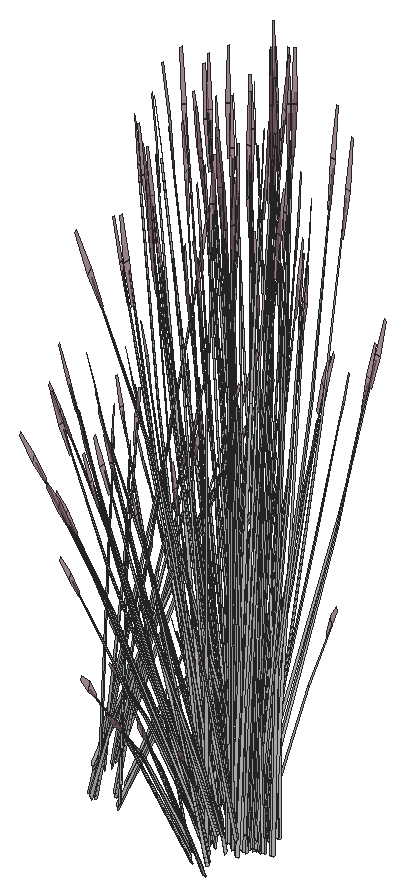
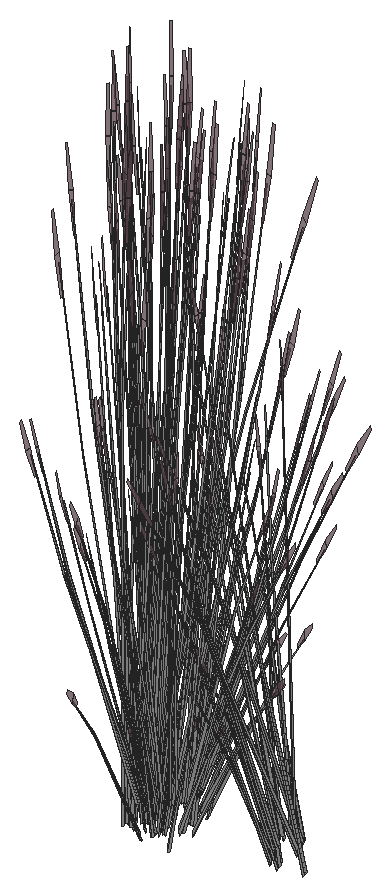
# SketchUp Ruby script. Lengths in inches.
U = 1.inch
M = Sketchup.active_model
def pt(a) = Geom::Point3d.new(a.map { |v| v * U })
def face(e, loops, mat)
  f = e.add_face(loops[0].map { |a| pt(a) })
  loops[1..].each { |l| e.add_face(l.map { |a| pt(a) }).erase! }
  f.material = f.back_material = mat if mat
  f
end
# faces: each face lists its corners as indices into pts; further lists are holes
def faces(e, pts, list, mat = nil) = list.each { |f| face(e, (f[0].is_a?(Array) ? f : [f]).map { |l| l.map { |i| pts[i] } }, mat) }
# xy, xz, yz: faces in a plane at the given z, y or x. An outline is a flat list of corners, or four numbers for a rectangle; further outlines are holes
def ring(l) = l.size == 4 ? [[l[0], l[1]], [l[2], l[1]], [l[2], l[3]], [l[0], l[3]]] : l.each_slice(2).to_a
def flat(e, list, mat, &to3) = list.each { |f| face(e, (f[0].is_a?(Array) ? f : [f]).map { |l| ring(l).map { |u, v| to3.(u, v) } }, mat) }
def xy(e, z, list, mat = nil) = flat(e, list, mat) { |x, y| [x, y, z] }
def xz(e, y, list, mat = nil) = flat(e, list, mat) { |x, z| [x, y, z] }
def yz(e, x, list, mat = nil) = flat(e, list, mat) { |y, z| [x, y, z] }
def lines(e, pts, list) = list.each { |a, b| e.add_line(pt(pts[a]), pt(pts[b])) }
# prism: a flat outline (further loops are holes) pulled along v
def prism(e, loops, v, mat = nil)
  f = face(e, loops, mat); d = Geom::Vector3d.new(v.map { |x| x * U })
  f.pushpull(f.normal.samedirection?(d) ? d.length : -d.length)
end
def box(e, o, s, mat = nil) = prism(e, [[o, [o[0] + s[0], o[1], o[2]], [o[0] + s[0], o[1] + s[1], o[2]], [o[0], o[1] + s[1], o[2]]]], [0, 0, s[2]], mat)
def at(x, y, z, deg = 0) = Geom::Transformation.translation(pt([x, y, z])) * Geom::Transformation.rotation(ORIGIN, Z_AXIS, deg.degrees)
def axes(o, x, y, z) = Geom::Transformation.new([*x, 0, *y, 0, *z, 0, *pt(o).to_a, 1])
def part(name) = M.definitions.add(name)
# library, detail: a bought-in or finely detailed component or shape, given as its bounding box
def library(name, o, s) = part(name).tap { |d| box(d.entities, o, s) }
def detail(e, o, s) = box(e.add_group.entities, o, s)
def put(e, d, t, mat = nil) = e.add_instance(d, t).tap { |i| i.material = mat if mat }
def group(e, t, mat = nil) = e.add_group.tap { |g| g.transformation = t; g.material = mat if mat }.entities
root = M.entities
M.materials.add("LightPink_Translucent").color = [144, 107, 117]
M.materials["LightPink_Translucent"].alpha = 0.75
M.materials.add("[_0053_Ivory_]").color = [200, 200, 200]
c1 = part("blade")
p = [[2.15,0.21,22],[0,0.17,0],[0.09,0.45,0],[2.18,0.31,22],[2.29,0.31,22],[0.38,0.45,0],
  [2.48,0.24,33],[2.49,0.24,33],[2.48,0.22,33]]
faces(c1.entities,p,[[0,1,2,3],[4,5,2,3],[6,3,4,7],[8,0,3,6]])
c2 = part("seeds")
p = [[0.3,-0.1,1.38],[-0.01,-0.03,1.59],[-0.01,-0.03,0.03],[0.14,-0.07,-0.07],[0.29,-0.03,3],[0.15,0.01,3.11]]
faces(c2.entities,p,[[0,1,2,3],[1,0,4,5]],"LightPink_Translucent")
c3 = part("blade with seeds")
put(c3.entities,c1,at(0,0,0))
put(c3.entities,c2,axes([2.4,0.25,30.99],[1.5799,-0.05474,1.17369],[-0.12525,1.92788,0.29478],[-0.07173,-0.02425,1.56792]))
put(root,c3,axes([471.34,101.96,128.71],[0.63179,0.1031,-0.62353],[-0.13332,0.63596,-0.16365],[0.18854,0.07706,1.37633]),"[_0053_Ivory_]")
put(root,c3,axes([481.84,101.41,130.53],[0.25192,-0.01424,1.71376],[-0.16712,0.61729,0.13857],[-0.35901,-0.03818,0.73262]),"[_0053_Ivory_]")
put(root,c3,axes([474.03,102.33,128.91],[-0.37654,-0.40212,-0.06488],[0.4124,-0.36845,-0.29416],[0.11685,-0.02594,0.97024]),"[_0053_Ivory_]")
put(root,c3,axes([473.17,100.29,129.42],[-0.2023,0.32011,1.1486],[-0.17388,-0.43009,0.84392],[0.16708,-0.10777,0.25299]),"[_0053_Ivory_]")
put(root,c3,axes([471.21,103.32,130.53],[-0.2256,-0.10835,1.71376],[0.46687,-0.45453,0.13857],[0.29098,0.20505,0.73262]),"[_0053_Ivory_]")
put(root,c3,axes([481.95,102.5,130.53],[0.21074,-0.13302,1.71376],[0.17741,0.61464,0.13857],[-0.33083,0.13891,0.73262]),"[_0053_Ivory_]")
put(root,c3,axes([472.88,101.49,131.18],[0.52868,-0.08987,-0.35414],[0.1396,0.51376,0.4572],[0.1515,-0.13799,0.87481]),"[_0053_Ivory_]")
put(root,c3,axes([481.29,103.54,129.24],[0.21107,0.05162,1.43002],[0.13604,0.52729,-0.30754],[-0.28671,0.0987,0.61141]),"[_0053_Ivory_]")
put(root,c3,axes([472.46,101.66,131.63],[0.31725,-0.49618,-0.71045],[0.55593,0.35263,0.08574],[0.18942,-0.17977,1.00501]),"[_0053_Ivory_]")
put(root,c3,axes([472.45,104.33,131.18],[0.34557,0.39372,-0.35414],[-0.39459,0.37271,0.4572],[0.20048,0.05671,0.87481]),"[_0053_Ivory_]")
put(root,c3,axes([483.16,101.86,130],[0.17264,-0.09097,1.77064],[0.05953,0.63516,0.13857],[-0.37394,0.08428,0.63284]),"[_0053_Ivory_]")
put(root,c3,axes([482.6,100.84,131.63],[-0.60713,-0.01514,-0.71045],[0.04078,-0.63759,0.08574],[-0.25721,-0.06729,1.00501]),"[_0053_Ivory_]")
put(root,c3,axes([482.11,100.99,129.24],[0.11858,0.17508,1.43002],[-0.27325,0.4759,-0.30754],[-0.28057,-0.11375,0.61141]),"[_0053_Ivory_]")
put(root,c3,axes([472.72,102.71,131.33],[0.16454,-0.57202,-0.51099],[0.56413,0.19607,-0.3958],[0.22713,-0.05245,0.97773]),"[_0053_Ivory_]")
put(root,c3,axes([474.14,103.07,129.42],[-0.37526,0.10382,1.1486],[0.17664,-0.42906,0.84392],[0.19907,0.02936,0.25299]),"[_0053_Ivory_]")
put(root,c3,axes([481.625,101.94,131.18],[-0.50475,-0.17543,-0.35414],[0.14722,-0.5118,0.4572],[-0.20322,0.04693,0.87481]),"[_0053_Ivory_]")
put(root,c3,axes([482.32,100.42,130.53],[0.2256,0.10835,1.71376],[-0.46687,0.45453,0.13857],[-0.29098,-0.20505,0.73262]),"[_0053_Ivory_]")
put(root,c3,axes([472.92,101.21,129.24],[-0.21697,-0.01863,1.43002],[-0.22228,-0.49966,-0.30754],[0.26655,-0.14135,0.61141]),"[_0053_Ivory_]")
put(root,c3,axes([473.06,102.97,131.18],[0.50475,0.17543,-0.35414],[-0.14722,0.5118,0.4572],[0.20322,-0.04693,0.87481]),"[_0053_Ivory_]")
put(root,c3,axes([481.97,102.2,131.33],[-0.16454,0.57202,-0.51099],[-0.56413,-0.19607,-0.3958],[-0.22713,0.05245,0.97773]),"[_0053_Ivory_]")
put(root,c3,axes([472.09,104.07,131.63],[0.60713,0.01514,-0.71045],[-0.04078,0.63759,0.08574],[0.25721,0.06729,1.00501]),"[_0053_Ivory_]")
put(root,c3,axes([482.4,100.97,131.33],[-0.44101,0.41656,-0.51099],[-0.38623,-0.44004,-0.3958],[-0.22407,-0.06338,0.97773]),"[_0053_Ivory_]")
put(root,c3,axes([481.6875,102.17,128.15],[0.0154,0.09911,1.76342],[-0.31051,0.51756,-0.26939],[-0.22056,-0.02609,0.30037]),"[_0053_Ivory_]")
put(root,c3,axes([473.32,102.87,128.64],[-0.39118,0.07547,1.41583],[-0.06226,-0.6007,0.08104],[0.27398,-0.09092,0.80566]),"[_0053_Ivory_]")
put(root,c3,axes([473.75,102.47,128.15],[-0.03174,-0.09547,1.76342],[0.22015,-0.55846,-0.26939],[0.22208,-0.00803,0.30037]),"[_0053_Ivory_]")
put(root,c3,axes([471.6875,102.33,130.53],[-0.25192,0.01424,1.71376],[0.16712,-0.61729,0.13857],[0.35901,0.03818,0.73262]),"[_0053_Ivory_]")
put(root,c3,axes([480.85,104.65,129.42],[0.25312,-0.28501,1.1486],[0.09988,0.45119,0.84392],[-0.18292,0.08079,0.25299]),"[_0053_Ivory_]")
put(root,c3,axes([472.61,102.91,131.63],[0.53369,-0.27773,-0.71045],[0.29743,0.5717,0.08574],[0.25786,-0.06494,1.00501]),"[_0053_Ivory_]")
put(root,c3,axes([482.23,100.57,131.18],[-0.34557,-0.39372,-0.35414],[0.39459,-0.37271,0.4572],[-0.20048,-0.05671,0.87481]),"[_0053_Ivory_]")
put(root,c3,axes([482.72,102.91,130.53],[0.1517,-0.19322,1.71376],[0.38303,0.52154,0.13857],[-0.26271,0.23751,0.73262]),"[_0053_Ivory_]")
put(root,c3,axes([481.81,103.42,131.18],[-0.52868,0.08987,-0.35414],[-0.1396,-0.51376,0.4572],[-0.1515,0.13799,0.87481]),"[_0053_Ivory_]")
put(root,c3,axes([481.52,104.94,128.15],[0.08147,0.06283,1.76342],[0.13814,0.58211,-0.26939],[-0.18056,0.12413,0.30037]),"[_0053_Ivory_]")
put(root,c3,axes([481.4,101.52,129.42],[0.38775,-0.045,1.1486],[-0.24596,0.39648,0.84392],[-0.19161,-0.05948,0.25299]),"[_0053_Ivory_]")
put(root,c3,axes([473.43,103.76,129.24],[-0.14627,-0.15466,1.43002],[0.19032,-0.51164,-0.30754],[0.29594,0.06931,0.61141]),"[_0053_Ivory_]")
put(root,c3,axes([482.61,103.39,130.53],[0.11309,-0.21615,1.71376],[0.47441,0.44731,0.13857],[-0.21402,0.27879,0.73262]),"[_0053_Ivory_]")
put(root,c3,axes([482.24,103.48,131.33],[0.15602,0.5742,-0.51099],[-0.59087,0.10045,-0.3958],[-0.16933,0.15423,0.97773]),"[_0053_Ivory_]")
put(root,c3,axes([483.72,103.06,128.71],[-0.63179,-0.1031,-0.62353],[0.13332,-0.63596,-0.16365],[-0.18854,-0.07706,1.37633]),"[_0053_Ivory_]")
put(root,c3,axes([483.65,100.09,131.63],[-0.51789,-0.30395,-0.71045],[0.36805,-0.53263,0.08574],[-0.18764,-0.18149,1.00501]),"[_0053_Ivory_]")
put(root,c3,axes([483.41,100.1,131.33],[-0.59932,0.14948,-0.51099],[-0.10484,-0.56611,-0.3958],[-0.16097,-0.16223,0.97773]),"[_0053_Ivory_]")
put(root,c3,axes([482.89,104.27,128.67],[-0.56842,-0.31443,-0.49651],[0.33976,-0.56381,0],[-0.12946,-0.07161,1.57504]),"[_0053_Ivory_]")
put(root,c3,axes([482.64,99.59,128.15],[-0.05883,0.08284,1.76342],[-0.59454,0.17861,-0.26939],[-0.14363,-0.16248,0.30037]),"[_0053_Ivory_]")
put(root,c3,axes([483.23,104.65,129.03],[-0.37973,0.63014,0],[-0.6353,-0.35142,-0.51607],[-0.14469,-0.08004,1.63711]),"[_0053_Ivory_]")
put(root,c3,axes([482.54,105.5625,129.24],[0.19166,-0.0992,1.43002],[0.4732,0.29912,-0.30754],[-0.14084,0.25882,0.61141]),"[_0053_Ivory_]")
put(root,c3,axes([482.27,99.9,128.78],[-0.1752,0.51349,-0.03893],[-0.53924,-0.15795,-0.17649],[-0.08187,-0.08399,0.58215]),"[_0053_Ivory_]")
put(root,c3,axes([483.07,99.26,129.24],[-0.03678,0.20572,1.43002],[-0.53767,0.17221,-0.30754],[-0.12568,-0.26589,0.61141]),"[_0053_Ivory_]")
put(root,c3,axes([483.25,99.79,130.53],[0.13883,0.2019,1.71376],[-0.64153,0.16998,0.13857],[-0.14499,-0.31697,0.73262]),"[_0053_Ivory_]")
put(root,c3,axes([484.43,103.16,129.32],[-0.61322,0.4175,-0.29095],[-0.40778,-0.58992,-0.50002],[-0.1513,-0.05991,1.59708]),"[_0053_Ivory_]")
put(root,c3,axes([483.47,99.68,131.18],[-0.0938,-0.50652,-0.35414],[0.53623,-0.13375,0.4572],[-0.14403,-0.14515,0.87481]),"[_0053_Ivory_]")
put(root,c3,axes([481.98,102.25,129.03],[-0.75945,0,0],[0,-0.70283,-0.51607],[0,-0.16007,1.63711]),"[_0053_Ivory_]")
put(root,c3,axes([483.05,104.03,128.68],[-0.14267,-0.54795,-0.30978],[0.56663,-0.1556,0.30978],[-0.11423,-0.06319,1.38974]),"[_0053_Ivory_]")
put(root,c3,axes([482.74,104.61,131.18],[-0.41095,0.33109,-0.35414],[-0.38901,-0.37805,0.4572],[-0.05919,0.19208,0.87481]),"[_0053_Ivory_]")
put(root,c3,axes([484.84,103.61,128.71],[-0.40909,0.47266,-0.62353],[-0.50819,-0.4286,-0.16365],[-0.16393,0.11791,1.37633]),"[_0053_Ivory_]")
put(root,c3,axes([482.57,102.0625,128.98],[-0.56493,0.5287,0.30756],[-0.56528,-0.52313,-0.36492],[-0.01973,-0.15014,1.64885]),"[_0053_Ivory_]")
put(root,c3,axes([484.89,103.52,129.98],[0.52485,0.25358,1.51261],[-0.51417,0.54629,0.59816],[-0.23031,-0.32378,1.26806]),"[_0053_Ivory_]")
put(root,c3,axes([482.89,98.93,129.42],[0.31682,0.21887,1.1486],[-0.4614,0.13157,0.84392],[-0.09872,-0.16821,0.25299]),"[_0053_Ivory_]")
put(root,c3,axes([485.12,103.35,129.12],[-0.59306,-0.50614,-0.25192],[0.49904,-0.56836,0.5513],[-0.1597,0.05921,1.68216]),"[_0053_Ivory_]")
put(root,c3,axes([484.04,102.86,128.86],[-0.36485,-0.52782,-0.44739],[0.55265,-0.37168,0.21531],[-0.11807,-0.06531,1.43643]),"[_0053_Ivory_]")
put(root,c3,axes([483.01,104.26,131.99],[-0.0158,0.58168,-0.7886],[-0.66548,-0.03907,0.09517],[-0.07023,0.24643,1.11556]),"[_0053_Ivory_]")
put(root,c3,axes([483,105.89,129.42],[-0.01572,-0.37392,1.1486],[0.39276,0.26669,0.84392],[-0.07724,0.17822,0.25299]),"[_0053_Ivory_]")
put(root,c3,axes([484.82,103.24,128.86],[-0.65953,0.03882,-0.44739],[-0.05964,-0.64439,0.21531],[-0.11807,0.06531,1.43643]),"[_0053_Ivory_]")
put(root,c3,axes([483.5625,104.32,129.13],[0.56842,0.31443,0.49651],[-0.33976,0.56381,0],[-0.12946,-0.07161,1.57504]),"[_0053_Ivory_]")
put(root,c3,axes([482.79,105.08,130.02],[0.01334,-0.32463,1.54345],[0.60018,0.17147,0.21329],[-0.052,0.34598,0.72882]),"[_0053_Ivory_]")
put(root,c3,axes([484.1,103.17,129.09],[0.16098,-0.74515,-0.23429],[0.76326,0.12989,0.51271],[-0.13337,-0.1029,1.5644]),"[_0053_Ivory_]")
put(root,c3,axes([484.375,103.34,129.27],[-0.11717,0.56122,0.1448],[-0.57245,-0.09742,-0.41347],[-0.10418,-0.05763,1.26744]),"[_0053_Ivory_]")
put(root,c3,axes([485.51,104.9,128.67],[-0.56842,0.31443,-0.49651],[-0.33976,-0.56381,0],[-0.12946,0.07161,1.57504]),"[_0053_Ivory_]")
put(root,c3,axes([482.15,101.77,128.67],[0,-0.62885,-0.49651],[0.67951,0,0],[0,-0.14322,1.57504]),"[_0053_Ivory_]")
put(root,c3,axes([482.44,102.36,129.13],[0,0.62885,0.49651],[-0.67951,0,0],[0,-0.14322,1.57504]),"[_0053_Ivory_]")
put(root,c3,axes([485.55,104.74,128.85],[-0.37499,-0.63235,-0.05142],[0.6353,-0.35142,0.51607],[-0.15655,0.0602,1.6363]),"[_0053_Ivory_]")
put(root,c3,axes([483.15,104.45,131.66],[0.43478,0.42253,-0.5672],[-0.45929,0.37004,-0.43934],[-0.06615,0.21468,1.08528]),"[_0053_Ivory_]")
put(root,c3,axes([485.38,104.66,128.68],[-0.56663,-0.1556,-0.30978],[0.14267,-0.54795,0.30978],[-0.11423,0.06319,1.38974]),"[_0053_Ivory_]")
put(root,c3,axes([483.93,102.5,129.32],[-0.68399,-0.30005,-0.29095],[0.32934,-0.63331,-0.50002],[-0.0215,-0.15549,1.59708]),"[_0053_Ivory_]")
put(root,c3,axes([485.71,102.3125,129.5],[-0.01659,-0.59209,1.41272],[0.75089,0.15348,0.59816],[-0.1776,0.32398,1.3335]),"[_0053_Ivory_]")
put(root,c3,axes([482.67,105.08,129.48],[0.55175,-0.11136,0.06507],[0.12684,0.44864,-0.86304],[-0.03498,0.22711,0.7736]),"[_0053_Ivory_]")
put(root,c3,axes([485.28,103.07,129.32],[0.07077,0.71755,-0.29095],[-0.73712,0.04339,-0.50002],[-0.1298,0.09558,1.59708]),"[_0053_Ivory_]")
put(root,c3,axes([483.62,101.86,128.75],[-0.24943,-0.64486,-0.69835],[0.71849,-0.23224,-0.18329],[-0.02757,-0.21836,1.54149]),"[_0053_Ivory_]")
put(root,c3,axes([484.74,99.84,131.33],[-0.59704,-0.15764,-0.51099],[0.20464,-0.54049,-0.3958],[-0.05475,-0.21761,0.97773]),"[_0053_Ivory_]")
put(root,c3,axes([483.64,103.84,130.53],[-0.01487,-0.24136,1.71376],[0.64429,0.16012,0.13857],[-0.03985,0.34396,0.73262]),"[_0053_Ivory_]")
put(root,c3,axes([482.44,101.79,128.68],[0.42396,-0.39235,-0.30978],[0.42396,0.39235,0.30978],[0,-0.12637,1.38974]),"[_0053_Ivory_]")
put(root,c3,axes([484.36,99.25,128.78],[-0.4197,0.36076,-0.03893],[-0.38456,-0.39511,-0.17649],[-0.02707,-0.11196,0.58215]),"[_0053_Ivory_]")
put(root,c3,axes([484.1875,102.81,129.01],[0.76764,0.13249,0.45755],[-0.15622,0.74829,0.17955],[-0.11218,-0.07226,1.58856]),"[_0053_Ivory_]")
put(root,c3,axes([483.99,102.67,129.37],[-0.29468,0.56664,0.44739],[-0.61229,-0.27271,-0.21531],[0,-0.13062,1.43643]),"[_0053_Ivory_]")
put(root,c3,axes([484.96,99.94,131.63],[-0.28988,-0.51132,-0.71045],[0.59671,-0.28496,0.08574],[-0.06778,-0.24706,1.00501]),"[_0053_Ivory_]")
put(root,c3,axes([483.77,104,129.13],[0.65264,-0.16691,0.17642],[0.16115,0.62115,0.35086],[-0.05821,-0.0905,1.60407]),"[_0053_Ivory_]")
put(root,c3,axes([484.61,104.1,128.85],[-0.61229,-0.28233,0],[0.29468,-0.58663,0],[0,0,1.62707]),"[_0053_Ivory_]")
put(root,c3,axes([486.03,104.81,129.03],[0.37973,0.63014,0],[-0.6353,0.35142,-0.51607],[-0.14469,0.08004,1.63711]),"[_0053_Ivory_]")
put(root,c3,axes([485.72,104.04,129.13],[0.17545,-0.62497,0.17642],[0.64204,0.17686,0.35086],[-0.11091,0.00304,1.60407]),"[_0053_Ivory_]")
put(root,c3,axes([485.42,103.21,129.27],[0.44871,0.37783,0.1448],[-0.37428,0.42627,-0.41347],[-0.10418,0.05763,1.26744]),"[_0053_Ivory_]")
put(root,c3,axes([485.26,102.74,128.95],[-0.56493,-0.54126,-0.06131],[0.56528,-0.54159,0],[-0.01973,-0.0189,1.75571]),"[_0053_Ivory_]")
put(root,c3,axes([485.41,102.93,129.37],[0.65953,-0.03882,0.44739],[0.05964,0.64439,-0.21531],[-0.11807,0.06531,1.43643]),"[_0053_Ivory_]")
put(root,c3,axes([485.57,104.41,128.98],[0.76036,0.2044,0.30756],[-0.19023,0.7306,-0.36492],[-0.12585,0.09144,1.64885]),"[_0053_Ivory_]")
put(root,c3,axes([484.46,98.81,128.15],[-0.10187,0.02266,1.76342],[-0.56336,-0.25503,-0.26939],[0.00945,-0.21273,0.30037]),"[_0053_Ivory_]")
put(root,c3,axes([485.9,104.37,129.13],[0.56842,-0.31443,0.49651],[0.33976,0.56381,0],[-0.12946,0.07161,1.57504]),"[_0053_Ivory_]")
put(root,c3,axes([485.02,99.51,131.18],[0.1831,-0.48359,-0.35414],[0.53419,0.14105,0.4572],[-0.04898,-0.1947,0.87481]),"[_0053_Ivory_]")
put(root,c3,axes([484.12,102.12,129.01],[0.26406,0.70318,0.45755],[-0.7545,0.24452,0.17955],[0.00922,-0.12921,1.58856]),"[_0053_Ivory_]")
put(root,c3,axes([484,102.03,128.86],[0.29468,-0.56664,-0.44739],[0.61229,0.27271,0.21531],[0,-0.13062,1.43643]),"[_0053_Ivory_]")
put(root,c3,axes([484.75,103.86,128.86],[-0.19817,-0.54216,0],[0.56587,-0.18986,0],[0,0,1.54371]),"[_0053_Ivory_]")
put(root,c3,axes([484.03,105,128.15],[0.09829,-0.03422,1.76342],[0.59126,0.18834,-0.26939],[0.01729,0.21228,0.30037]),"[_0053_Ivory_]")
put(root,c3,axes([484.16,105.19,131.18],[-0.1831,0.48359,-0.35414],[-0.53419,-0.14105,0.4572],[0.04898,0.1947,0.87481]),"[_0053_Ivory_]")
put(root,c3,axes([485.55,102.79,128.86],[-0.29468,0.56664,-0.44739],[-0.61229,-0.27271,0.21531],[0,0.13062,1.43643]),"[_0053_Ivory_]")
put(root,c3,axes([486.72,102.44,129.13],[-0.47719,-0.45806,0.17642],[0.48088,-0.44429,0.35086],[-0.0527,0.09355,1.60407]),"[_0053_Ivory_]")
put(root,c3,axes([485.07,102.18,128.86],[0,-0.72763,0],[0.75945,0,0],[0,0,1.79456]),"[_0053_Ivory_]")
put(root,c3,axes([484.36,102.31,129.09],[0.68433,0.30479,0.24065],[-0.32934,0.63331,0.50002],[0,-0.14599,1.60543]),"[_0053_Ivory_]")
put(root,c3,axes([485.45,102.47,128.95],[0,0.72727,-0.05637],[-0.75945,0,0],[0,0.02286,1.79368]),"[_0053_Ivory_]")
put(root,c3,axes([484.14,101.89,129.37],[-0.65953,0.03882,0.44739],[-0.05964,-0.64439,-0.21531],[0.11807,-0.06531,1.43643]),"[_0053_Ivory_]")
put(root,c3,axes([483.84,100.78,129.13],[-0.17545,0.62497,0.17642],[-0.64204,-0.17686,0.35086],[0.11091,-0.00304,1.60407]),"[_0053_Ivory_]")
put(root,c3,axes([485.09,103.875,128.94],[0.26406,0.72244,-0.06012],[-0.7545,0.25315,0],[0.00922,0.02523,1.72173]),"[_0053_Ivory_]")
put(root,c3,axes([483.52,100.01,129.03],[-0.37973,-0.63014,0],[0.6353,-0.35142,-0.51607],[0.14469,-0.08004,1.63711]),"[_0053_Ivory_]")
put(root,c3,axes([484.22,104.76,131.63],[0.28988,0.51132,-0.71045],[-0.59671,0.28496,0.08574],[0.06778,0.24706,1.00501]),"[_0053_Ivory_]")
put(root,c3,axes([487.27,102.93,128.85],[-0.75908,-0.00503,-0.04976],[0,-0.70283,0.49943],[-0.02386,0.16,1.58352]),"[_0053_Ivory_]")
put(root,c3,axes([485.78,100.8125,129.13],[-0.65264,0.16691,0.17642],[-0.16115,-0.62115,0.35086],[0.05821,0.0905,1.60407]),"[_0053_Ivory_]")
put(root,c3,axes([485.11,98.48,129.42],[0.07791,0.3667,1.1486],[-0.43222,-0.2031,0.84392],[0.04651,-0.18776,0.25299]),"[_0053_Ivory_]")
put(root,c3,axes([484.71,101.72,129.01],[-0.50358,0.57069,0.45755],[-0.59827,-0.50377,0.17955],[0.1214,-0.05695,1.58856]),"[_0053_Ivory_]")
put(root,c3,axes([485.57,102.62,128.87],[0.42396,0.40619,0],[-0.42396,0.40619,0],[0,0,1.69266]),"[_0053_Ivory_]")
put(root,c3,axes([485.56,102.14,129.37],[0.29468,-0.56664,0.44739],[0.61229,0.27271,-0.21531],[0,0.13062,1.43643]),"[_0053_Ivory_]")
put(root,c3,axes([485.31,104.11,128.86],[0.61229,0.28233,0],[-0.29468,0.58663,0],[0,0,1.74954]),"[_0053_Ivory_]")
put(root,c3,axes([484.4375,104.86,131.33],[0.59704,0.15764,-0.51099],[-0.20464,0.54049,-0.3958],[0.05475,0.21761,0.97773]),"[_0053_Ivory_]")
put(root,c3,axes([485.37,102.01,129.03],[-0.76764,-0.13249,0.49198],[0.15622,-0.74829,0.19306],[0.11218,0.07226,1.70813]),"[_0053_Ivory_]")
put(root,c3,axes([487.11,103.03,128.68],[-0.42396,0.39235,-0.30978],[-0.42396,-0.39235,0.30978],[0,0.12637,1.38974]),"[_0053_Ivory_]")
put(root,c3,axes([485.9,102.96,128.75],[0.2227,0.57576,-0.69212],[-0.64151,0.20736,-0.18165],[0.02462,0.19497,1.52773]),"[_0053_Ivory_]")
put(root,c3,axes([485.59,102.34,128.86],[0.67951,0,0],[0,0.65103,0],[0,0,1.78407]),"[_0053_Ivory_]")
put(root,c3,axes([484.93,101.62,129.37],[-0.36485,-0.52782,0.44739],[0.55265,-0.37168,-0.21531],[0.11807,0.06531,1.43643]),"[_0053_Ivory_]")
put(root,c3,axes([484.27,101.75,129.32],[-0.07077,-0.71755,-0.29095],[0.73712,-0.04339,-0.50002],[0.1298,-0.09558,1.59708]),"[_0053_Ivory_]")
put(root,c3,axes([485.82,102.27,129.27],[0.56587,-0.18339,0.1448],[0.19817,0.52368,-0.41347],[0,0.11525,1.26744]),"[_0053_Ivory_]")
put(root,c3,axes([486.03,100.25,131.33],[-0.43478,-0.42253,-0.51099],[0.45929,-0.37004,-0.3958],[0.06615,-0.21468,0.97773]),"[_0053_Ivory_]")
put(root,c3,axes([485.625,102.32,129.32],[0.68399,0.30005,-0.29095],[-0.32934,0.63331,-0.50002],[0.0215,0.15549,1.59708]),"[_0053_Ivory_]")
